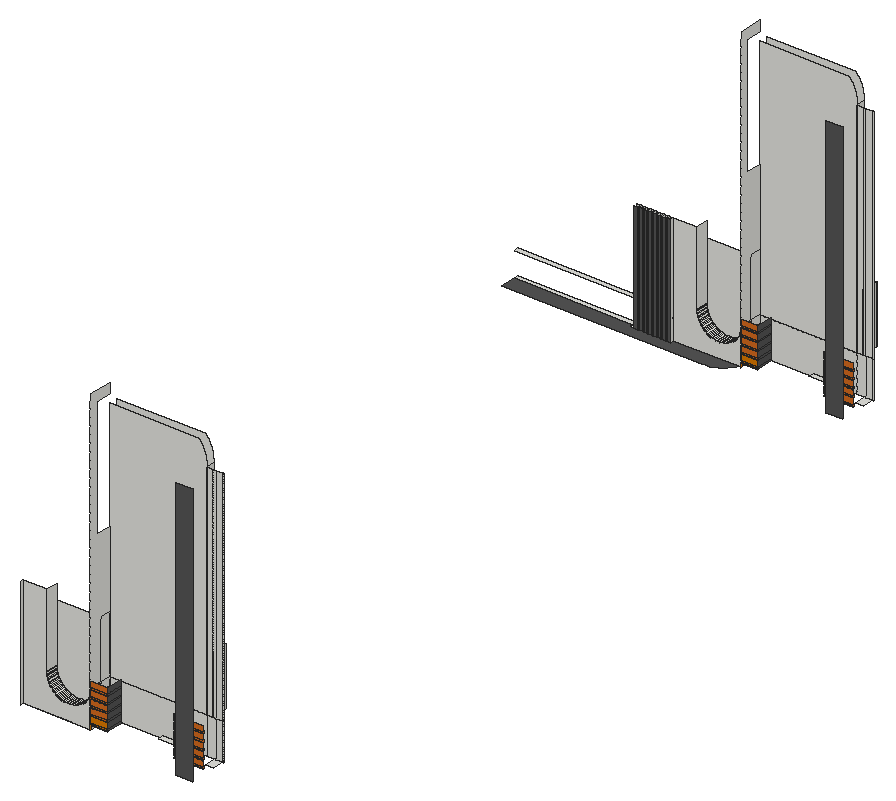
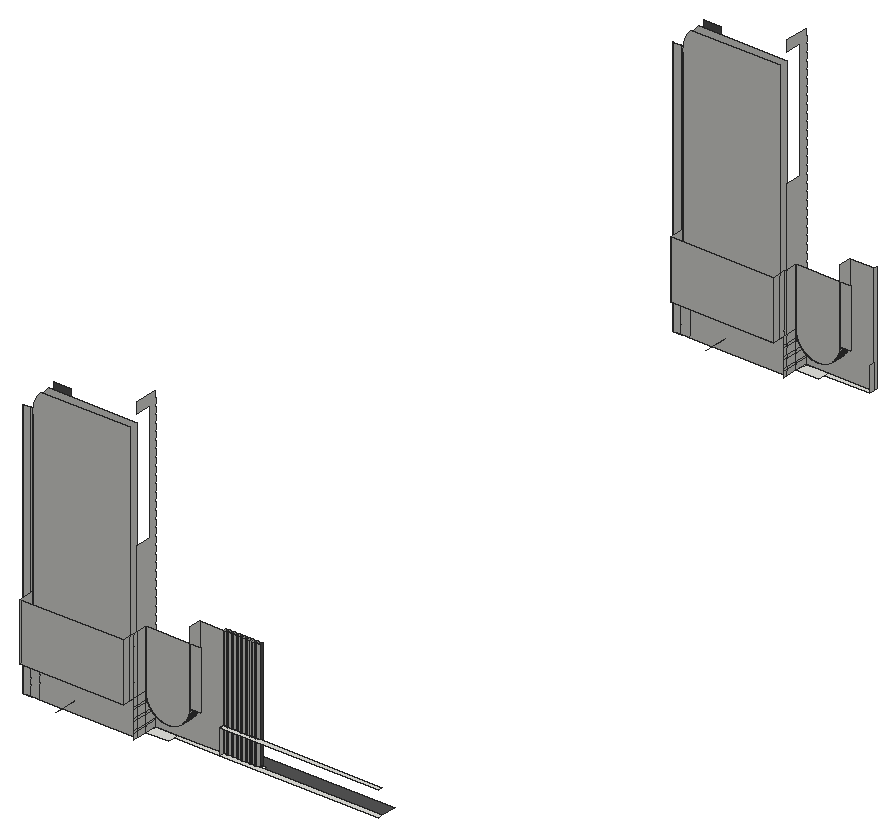
# SketchUp Ruby script. Lengths in inches.
U = 1.inch
M = Sketchup.active_model
def pt(a) = Geom::Point3d.new(a.map { |v| v * U })
def face(e, loops, mat)
  f = e.add_face(loops[0].map { |a| pt(a) })
  loops[1..].each { |l| e.add_face(l.map { |a| pt(a) }).erase! }
  f.material = f.back_material = mat if mat
  f
end
# faces: each face lists its corners as indices into pts; further lists are holes
def faces(e, pts, list, mat = nil) = list.each { |f| face(e, (f[0].is_a?(Array) ? f : [f]).map { |l| l.map { |i| pts[i] } }, mat) }
# xy, xz, yz: faces in a plane at the given z, y or x. An outline is a flat list of corners, or four numbers for a rectangle; further outlines are holes
def ring(l) = l.size == 4 ? [[l[0], l[1]], [l[2], l[1]], [l[2], l[3]], [l[0], l[3]]] : l.each_slice(2).to_a
def flat(e, list, mat, &to3) = list.each { |f| face(e, (f[0].is_a?(Array) ? f : [f]).map { |l| ring(l).map { |u, v| to3.(u, v) } }, mat) }
def xy(e, z, list, mat = nil) = flat(e, list, mat) { |x, y| [x, y, z] }
def xz(e, y, list, mat = nil) = flat(e, list, mat) { |x, z| [x, y, z] }
def yz(e, x, list, mat = nil) = flat(e, list, mat) { |y, z| [x, y, z] }
def lines(e, pts, list) = list.each { |a, b| e.add_line(pt(pts[a]), pt(pts[b])) }
# prism: a flat outline (further loops are holes) pulled along v
def prism(e, loops, v, mat = nil)
  f = face(e, loops, mat); d = Geom::Vector3d.new(v.map { |x| x * U })
  f.pushpull(f.normal.samedirection?(d) ? d.length : -d.length)
end
def box(e, o, s, mat = nil) = prism(e, [[o, [o[0] + s[0], o[1], o[2]], [o[0] + s[0], o[1] + s[1], o[2]], [o[0], o[1] + s[1], o[2]]]], [0, 0, s[2]], mat)
def at(x, y, z, deg = 0) = Geom::Transformation.translation(pt([x, y, z])) * Geom::Transformation.rotation(ORIGIN, Z_AXIS, deg.degrees)
def axes(o, x, y, z) = Geom::Transformation.new([*x, 0, *y, 0, *z, 0, *pt(o).to_a, 1])
def part(name) = M.definitions.add(name)
# library, detail: a bought-in or finely detailed component or shape, given as its bounding box
def library(name, o, s) = part(name).tap { |d| box(d.entities, o, s) }
def detail(e, o, s) = box(e.add_group.entities, o, s)
def put(e, d, t, mat = nil) = e.add_instance(d, t).tap { |i| i.material = mat if mat }
def group(e, t, mat = nil) = e.add_group.tap { |g| g.transformation = t; g.material = mat if mat }.entities
root = M.entities
M.materials.add("[0039_DarkOrange]").color = [219, 120, 0]
M.materials.add("[0041_Chocolate]").color = [210, 105, 30]
M.materials.add("[Color M06]").color = [84, 84, 84]
xy(root,141.26,[[2137,281.47,2177.59,285.84],[2177.59,281.47,2195.57,281.47,2196.33,283,2197.37,286.06,2198,289.23,2198.21,292.45,2177.59,292.45],[2195.57,281.47,2196.33,283,2197.37,286.06,2198,289.23,2198.21,292.45,2198.21,281.47],[2292.85,292.45,2299.64,302.46],[2026.42,972.36,2169.44,976.74],
  [2169.44,972.36,2210.03,976.74],[2210.03,972.36,2228.01,972.36,2228.77,973.89,2229.81,976.95,2230.4375,980.12,2230.65,983.34,2210.03,983.34],[2228.01,972.36,2228.77,973.89,2229.81,976.95,2230.4375,980.12,2230.65,983.34,2230.65,972.36],[2325.29,983.34,2332.08,993.35]])
xy(root,141.26,[[2026.42,958.64,2205.95,958.64,2209.17,958.86,2212.34,959.49,2215.4,960.52,2218.3,961.95,2220.98,963.75,2223.41,965.88,2225.54,968.31,2227.34,970.99,2228.01,972.36,2169.44,972.36,2169.44,969.24,2166.32,969.24,2166.32,972.36,2165.07,972.36,2165.07,969.24,2161.94,969.24,2161.94,972.36,2160.88,972.36,2160.88,969.24,2157.75,969.24,2157.75,972.36,2156.69,972.36,2156.69,969.24,2153.57,969.24,2153.57,972.36,2152.5,972.36,2152.5,969.24,2149.38,969.24,2149.38,972.36,2148.32,972.36,2148.32,969.24,2145.19,969.24,2145.19,972.36,2144.07,972.36,2144.07,969.24,2140.94,969.24,2140.94,972.36,2139.82,972.36,2139.82,969.24,2136.69,969.24,2136.69,972.36,2135.57,972.36,2135.57,969.24,2132.44,969.24,2132.44,972.36,2026.42,972.36]],"[Color M06]")
xy(root,145.27,[[2247.98,295.65,2273.17,300.34],[2280.42,986.55,2305.61,991.24]])
xy(root,145.27,[[2198.21,280.47,2213.6,281.47],[2230.65,971.36,2246.03,972.36]],"[0039_DarkOrange]")
xy(root,145.27,[[2273.17,280.47,2299.64,281.47],[2305.61,971.36,2332.08,972.36]],"[0041_Chocolate]")
xy(root,147.375,[[2198.21,280.47,2213.6,281.47],[2230.65,971.36,2246.03,972.36]],"[0039_DarkOrange]")
xy(root,147.375,[[2273.17,280.47,2299.64,281.47],[2305.61,971.36,2332.08,972.36]],"[0041_Chocolate]")
xy(root,152.33,[[2198.21,280.47,2213.6,281.47],[2230.65,971.36,2246.03,972.36]],"[0039_DarkOrange]")
xy(root,152.33,[[2273.17,280.47,2299.64,281.47],[2305.61,971.36,2332.08,972.36]],"[0041_Chocolate]")
xy(root,154.4375,[[2198.21,280.47,2213.6,281.47],[2273.17,280.47,2299.64,281.47],[2230.65,971.36,2246.03,972.36],[2305.61,971.36,2332.08,972.36]],"[0041_Chocolate]")
xy(root,159.39,[[2198.21,280.47,2213.6,281.47],[2273.17,280.47,2299.64,281.47],[2230.65,971.36,2246.03,972.36],[2305.61,971.36,2332.08,972.36]],"[0041_Chocolate]")
xy(root,161.5,[[2198.21,280.47,2213.6,281.47],[2273.17,280.47,2299.64,281.47],[2230.65,971.36,2246.03,972.36],[2305.61,971.36,2332.08,972.36]],"[0041_Chocolate]")
xy(root,163.7,[[2026.42,972.36,2169.44,976.74]])
xy(root,166.45,[[2198.21,280.47,2213.6,281.47],[2273.17,280.47,2299.64,281.47],[2230.65,971.36,2246.03,972.36],[2305.61,971.36,2332.08,972.36]],"[0041_Chocolate]")
xy(root,168.5625,[[2198.21,280.47,2213.6,281.47],[2273.17,280.47,2299.64,281.47],[2230.65,971.36,2246.03,972.36],[2305.61,971.36,2332.08,972.36]],"[0041_Chocolate]")
xy(root,173.52,[[2198.21,280.47,2213.6,281.47],[2273.17,280.47,2299.64,281.47],[2230.65,971.36,2246.03,972.36],[2305.61,971.36,2332.08,972.36]],"[0041_Chocolate]")
xy(root,174.51,[[2198.21,302.46,2285.18,310.27],[2285.18,302.46,2285.18,310.27,2198.21,310.27,2198.21,317.3125,2291.02,317.3125,2291.02,302.46],[2230.65,993.35,2317.62,1001.16],[2317.62,993.35,2317.62,1001.16,2230.65,1001.16,2230.65,1008.21,2323.46,1008.21,2323.46,993.35]])
xy(root,175.625,[[2198.21,280.47,2213.6,281.47],[2273.17,280.47,2299.64,281.47],[2230.65,971.36,2246.03,972.36],[2305.61,971.36,2332.08,972.36]],"[0041_Chocolate]")
xz(root,267.75,[[2285.18,141.3,2300.52,376.875]],"[Color M06]")
xz(root,280.47,[[2198.21,147.375,2213.6,152.33]],"[0039_DarkOrange]")
xz(root,280.47,[[2273.17,147.375,2299.64,152.33],[2198.21,154.4375,2213.6,159.39],[2273.17,154.4375,2299.64,159.39],[2198.21,161.5,2213.6,166.45],[2273.17,161.5,2299.64,166.45],
  [2198.21,168.5625,2213.6,173.52],[2273.17,168.5625,2299.64,173.52],[2198.21,175.625,2213.6,180.58],[2273.17,175.625,2299.64,180.58]],"[0041_Chocolate]")
xz(root,281.47,[[2137,141.26,2198.21,141.26,2198.21,174.51,2198.18,173.46,2198.1,172.42,2197.96,171.38,2197.77,170.36,2197.53,169.34,2197.23,168.33,2196.88,167.35,2196.48,166.38,2196.03,165.4375,2195.53,164.52,2194.99,163.625,2194.39,162.76,2193.76,161.93,2193.08,161.14,2192.36,160.38,2191.6,159.66,2190.8,158.98,2189.97,158.34,2189.11,157.75,2188.22,157.2,2187.3,156.7,2186.36,156.25,2185.39,155.85,2184.4,155.5,2183.4,155.21,2182.38,154.96,2181.35,154.77,2180.32,154.64,2179.27,154.55,2178.23,154.53,2177.18,154.55,2176.14,154.64,2175.1,154.77,2174.07,154.96,2173.05,155.21,2172.05,155.5,2171.07,155.85,2170.1,156.25,2169.15,156.7,2168.23,157.2,2167.34,157.75,2166.48,158.34,2165.65,158.98,2164.85,159.66,2164.1,160.38,2163.375,161.14,2162.7,161.93,2162.06,162.76,2161.47,163.625,2160.92,164.52,2160.42,165.4375,2159.97,166.38,2159.57,167.35,2159.22,168.33,2158.92,169.34,2158.68,170.36,2158.49,171.38,2158.35,172.42,2158.27,173.46,2158.24,174.51,2158.24,240.16,2137,240.16]])
xz(root,281.47,[[2198.21,145.27,2213.6,147.375]],"[0039_DarkOrange]")
xz(root,281.47,[[2273.17,145.27,2299.64,147.375],[2198.21,152.33,2213.6,154.4375],[2273.17,152.33,2299.64,154.4375],[2198.21,159.39,2213.6,161.5],[2273.17,159.39,2299.64,161.5],
  [2198.21,166.45,2213.6,168.5625],[2273.17,166.45,2299.64,168.5625],[2198.21,173.52,2213.6,175.625],[2273.17,173.52,2299.64,175.625]],"[0041_Chocolate]")
xz(root,292.45,[[2178.23,154.53,2179.27,154.55,2180.32,154.64,2181.35,154.77,2182.38,154.96,2183.4,155.21,2184.4,155.5,2185.39,155.85,2186.36,156.25,2187.3,156.7,2188.22,157.2,2189.11,157.75,2189.97,158.34,2190.8,158.98,2191.6,159.66,2192.36,160.38,2193.08,161.14,2193.76,161.93,2194.39,162.76,2194.99,163.625,2195.53,164.52,2196.03,165.4375,2196.48,166.38,2196.88,167.35,2197.23,168.33,2197.53,169.34,2197.77,170.36,2197.96,171.38,2198.1,172.42,2198.18,173.46,2198.21,174.51,2198.21,226.8,2158.24,226.8,2158.24,174.51,2158.27,173.46,2158.35,172.42,2158.49,171.38,2158.68,170.36,2158.92,169.34,2159.22,168.33,2159.57,167.35,2159.97,166.38,2160.42,165.4375,2160.92,164.52,2161.47,163.625,2162.06,162.76,2162.7,161.93,2163.375,161.14,2164.1,160.38,2164.85,159.66,2165.65,158.98,2166.48,158.34,2167.34,157.75,2168.23,157.2,2169.15,156.7,2170.1,156.25,2171.07,155.85,2172.05,155.5,2173.05,155.21,2174.07,154.96,2175.1,154.77,2176.14,154.64,2177.18,154.55],[2148.59,174.51,2158.24,226.8]])
xz(root,302.46,[[2198.21,141.26,2285.18,174.51],[2285.18,141.26,2293.73,174.51],[2293.73,141.26,2299.64,174.51],[2299.64,141.26,2300.52,174.51],[2198.21,174.51,2285.18,174.51,2285.18,376.875,2285.17,377.55,2285.14,378.22,2285.1,378.9,2285.04,379.57,2284.96,380.24,2284.86,380.9,2284.75,381.57,2284.62,382.23,2284.47,382.89,2284.3,383.54,2284.28,383.64,2284.12,384.19,2283.92,384.84,2283.7,385.47,2283.6,385.76,2283.47,386.11,2283.22,386.73,2282.95,387.35,2282.67,387.96,2282.37,388.57,2282.06,389.17,2281.73,389.76,2281.38,390.33,2281.02,390.9,2280.65,391.47,2280.26,392.02,2279.86,392.56,2279.4375,393.09,2279.4,393.14,2279.01,393.6,2278.5625,394.11,2278.1,394.61,2277.63,395.09,2277.46,395.26,2198.21,395.26],
  [2285.18,174.51,2291.02,374.14],[2291.02,174.51,2293.73,374.14],[2293.73,174.51,2299.64,374.14],[2299.64,174.51,2300.52,374.14]])
xz(root,310.27,[[2198.21,174.51,2198.21,395.26,2277.46,395.26,2277.63,395.09,2278.1,394.61,2278.5625,394.11,2279.01,393.6,2279.4,393.14,2279.4375,393.09,2279.86,392.56,2280.26,392.02,2280.65,391.47,2281.02,390.9,2281.38,390.33,2281.73,389.76,2282.06,389.17,2282.37,388.57,2282.67,387.96,2282.95,387.35,2283.22,386.73,2283.47,386.11,2283.6,385.76,2283.7,385.47,2283.92,384.84,2284.12,384.19,2284.28,383.64,2284.3,383.54,2284.47,382.89,2284.62,382.23,2284.75,381.57,2284.86,380.9,2284.96,380.24,2285.04,379.57,2285.1,378.9,2285.14,378.22,2285.17,377.55,2285.18,376.875,2285.18,174.51]])
xz(root,317.3125,[[2198.21,174.51,2291.02,226.8]])
xz(root,958.64,[[2317.62,141.3,2332.96,376.875]],"[Color M06]")
xz(root,969.24,[[2136.69,141.26,2139.82,240.16],[2140.94,141.26,2144.07,240.16],[2145.19,141.26,2148.32,240.16],[2149.38,141.26,2152.5,240.16],[2153.57,141.26,2156.69,240.16],
  [2157.75,141.26,2160.88,240.16],[2161.94,141.26,2165.07,240.16],[2166.32,141.26,2169.44,240.16]],"[Color M06]")
xz(root,971.36,[[2230.65,147.375,2246.03,152.33]],"[0039_DarkOrange]")
xz(root,971.36,[[2305.61,147.375,2332.08,152.33],[2230.65,154.4375,2246.03,159.39],[2305.61,154.4375,2332.08,159.39],[2230.65,161.5,2246.03,166.45],[2305.61,161.5,2332.08,166.45],
  [2230.65,168.5625,2246.03,173.52],[2305.61,168.5625,2332.08,173.52],[2230.65,175.625,2246.03,180.58],[2305.61,175.625,2332.08,180.58]],"[0041_Chocolate]")
xz(root,972.36,[[2136.69,141.26,2139.82,163.7],[2139.82,141.26,2140.94,163.7],[2140.94,141.26,2144.07,163.7],[2144.07,141.26,2145.19,163.7],[2145.19,141.26,2148.32,163.7],
  [2148.32,141.26,2149.38,163.7],[2149.38,141.26,2152.5,163.7],[2152.5,141.26,2153.57,163.7],[2153.57,141.26,2156.69,163.7],[2156.69,141.26,2157.75,163.7],
  [2157.75,141.26,2160.88,163.7],[2160.88,141.26,2161.94,163.7],[2161.94,141.26,2165.07,163.7],[2165.07,141.26,2166.32,163.7],[2166.32,141.26,2169.44,163.7],
  [2169.44,141.26,2230.65,141.26,2230.65,174.51,2230.62,173.46,2230.54,172.42,2230.4,171.38,2230.21,170.36,2229.97,169.34,2229.67,168.33,2229.32,167.35,2228.92,166.38,2228.47,165.4375,2227.97,164.52,2227.42,163.625,2226.83,162.76,2226.19,161.93,2225.52,161.14,2224.8,160.38,2224.04,159.66,2223.24,158.98,2222.41,158.34,2221.55,157.75,2220.66,157.2,2219.74,156.7,2218.79,156.25,2217.83,155.85,2216.84,155.5,2215.84,155.21,2214.82,154.96,2213.79,154.77,2212.75,154.64,2211.71,154.55,2210.66,154.53,2209.62,154.55,2208.58,154.64,2207.54,154.77,2206.51,154.96,2205.49,155.21,2204.49,155.5,2203.5,155.85,2202.54,156.25,2201.59,156.7,2200.67,157.2,2199.78,157.75,2198.92,158.34,2198.09,158.98,2197.29,159.66,2196.53,160.38,2195.8125,161.14,2195.13,161.93,2194.5,162.76,2193.9,163.625,2193.36,164.52,2192.86,165.4375,2192.41,166.38,2192.01,167.35,2191.66,168.33,2191.36,169.34,2191.12,170.36,2190.93,171.38,2190.79,172.42,2190.71,173.46,2190.68,174.51,2190.68,240.16,2169.44,240.16],[2136.69,163.7,2139.82,240.16],[2140.94,163.7,2144.07,240.16],[2145.19,163.7,2148.32,240.16],[2149.38,163.7,2152.5,240.16],
  [2153.57,163.7,2156.69,240.16],[2157.75,163.7,2160.88,240.16],[2161.94,163.7,2165.07,240.16],[2166.32,163.7,2169.44,240.16]])
xz(root,972.36,[[2230.65,145.27,2246.03,147.375]],"[0039_DarkOrange]")
xz(root,972.36,[[2305.61,145.27,2332.08,147.375],[2230.65,152.33,2246.03,154.4375],[2305.61,152.33,2332.08,154.4375],[2230.65,159.39,2246.03,161.5],[2305.61,159.39,2332.08,161.5],
  [2230.65,166.45,2246.03,168.5625],[2305.61,166.45,2332.08,168.5625],[2230.65,173.52,2246.03,175.625],[2305.61,173.52,2332.08,175.625]],"[0041_Chocolate]")
xz(root,983.34,[[2210.66,154.53,2211.71,154.55,2212.75,154.64,2213.79,154.77,2214.82,154.96,2215.84,155.21,2216.84,155.5,2217.83,155.85,2218.79,156.25,2219.74,156.7,2220.66,157.2,2221.55,157.75,2222.41,158.34,2223.24,158.98,2224.04,159.66,2224.8,160.38,2225.52,161.14,2226.19,161.93,2226.83,162.76,2227.42,163.625,2227.97,164.52,2228.47,165.4375,2228.92,166.38,2229.32,167.35,2229.67,168.33,2229.97,169.34,2230.21,170.36,2230.4,171.38,2230.54,172.42,2230.62,173.46,2230.65,174.51,2230.65,226.8,2190.68,226.8,2190.68,174.51,2190.71,173.46,2190.79,172.42,2190.93,171.38,2191.12,170.36,2191.36,169.34,2191.66,168.33,2192.01,167.35,2192.41,166.38,2192.86,165.4375,2193.36,164.52,2193.9,163.625,2194.5,162.76,2195.13,161.93,2195.8125,161.14,2196.53,160.38,2197.29,159.66,2198.09,158.98,2198.92,158.34,2199.78,157.75,2200.67,157.2,2201.59,156.7,2202.54,156.25,2203.5,155.85,2204.49,155.5,2205.49,155.21,2206.51,154.96,2207.54,154.77,2208.58,154.64,2209.62,154.55],[2181.03,174.51,2190.68,226.8]])
xz(root,993.35,[[2230.65,141.26,2317.62,174.51],[2317.62,141.26,2326.17,174.51],[2326.17,141.26,2332.08,174.51],[2332.08,141.26,2332.96,174.51],[2230.65,174.51,2317.62,174.51,2317.62,376.875,2317.61,377.55,2317.58,378.22,2317.54,378.9,2317.48,379.57,2317.4,380.24,2317.3,380.9,2317.19,381.57,2317.05,382.23,2316.9,382.89,2316.74,383.54,2316.71,383.64,2316.56,384.19,2316.36,384.84,2316.14,385.47,2316.03,385.76,2315.91,386.11,2315.66,386.73,2315.39,387.35,2315.11,387.96,2314.81,388.57,2314.49,389.17,2314.17,389.76,2313.82,390.33,2313.46,390.9,2313.09,391.47,2312.7,392.02,2312.29,392.56,2311.875,393.09,2311.84,393.14,2311.44,393.6,2311,394.11,2310.54,394.61,2310.07,395.09,2309.9,395.26,2230.65,395.26],
  [2317.62,174.51,2323.46,374.14],[2323.46,174.51,2326.17,374.14],[2326.17,174.51,2332.08,374.14],[2332.08,174.51,2332.96,374.14]])
xz(root,1001.16,[[2230.65,174.51,2230.65,395.26,2309.9,395.26,2310.07,395.09,2310.54,394.61,2311,394.11,2311.44,393.6,2311.84,393.14,2311.875,393.09,2312.29,392.56,2312.7,392.02,2313.09,391.47,2313.46,390.9,2313.82,390.33,2314.17,389.76,2314.49,389.17,2314.81,388.57,2315.11,387.96,2315.39,387.35,2315.66,386.73,2315.91,386.11,2316.03,385.76,2316.14,385.47,2316.36,384.84,2316.56,384.19,2316.71,383.64,2316.74,383.54,2316.9,382.89,2317.05,382.23,2317.19,381.57,2317.3,380.9,2317.4,380.24,2317.48,379.57,2317.54,378.9,2317.58,378.22,2317.61,377.55,2317.62,376.875,2317.62,174.51]])
xz(root,1008.21,[[2230.65,174.51,2323.46,226.8]])
yz(root,2137,[[278.34,141.26,281.47,240.16],[281.47,141.26,285.84,163.7]])
yz(root,2139.82,[[969.24,141.26,972.36,240.16]])
yz(root,2140.94,[[969.24,141.26,972.36,240.16]])
yz(root,2144.07,[[969.24,141.26,972.36,240.16]])
yz(root,2145.19,[[969.24,141.26,972.36,240.16]])
yz(root,2148.32,[[969.24,141.26,972.36,240.16]])
yz(root,2149.38,[[969.24,141.26,972.36,240.16]])
yz(root,2152.5,[[969.24,141.26,972.36,240.16]])
yz(root,2153.57,[[969.24,141.26,972.36,240.16]])
yz(root,2156.69,[[969.24,141.26,972.36,240.16]])
yz(root,2157.75,[[969.24,141.26,972.36,240.16]])
yz(root,2158.24,[[281.47,174.51,292.45,240.16]])
yz(root,2160.88,[[969.24,141.26,972.36,240.16]])
yz(root,2161.94,[[969.24,141.26,972.36,240.16]])
yz(root,2165.07,[[969.24,141.26,972.36,240.16]])
yz(root,2166.32,[[969.24,141.26,972.36,240.16]])
yz(root,2169.44,[[969.24,141.26,972.36,240.16],[972.36,141.26,976.74,163.7]])
yz(root,2190.68,[[972.36,174.51,983.34,240.16]])
yz(root,2198.21,[[281.47,141.26,292.45,146.14],[292.45,141.26,302.46,146.14],[302.46,141.26,305.58,146.14],[281.47,146.14,292.45,148.26],[292.45,146.14,302.46,148.26],
  [302.46,146.14,305.58,148.26],[281.47,148.26,292.45,155.64],[292.45,148.26,302.46,155.64],[302.46,148.26,305.58,155.64],[281.47,155.64,292.45,157.76],
  [292.45,155.64,302.46,157.76],[302.46,155.64,305.58,157.76],[281.47,157.76,292.45,165.14],[292.45,157.76,302.46,165.14],[302.46,157.76,305.58,165.14],
  [281.47,165.14,292.45,167.26],[292.45,165.14,302.46,167.26],[302.46,165.14,305.58,167.26],[281.47,167.26,292.45,174.51],[292.45,167.26,302.46,174.51],
  [302.46,167.26,305.58,174.51],[281.47,174.51,281.47,175.625,280.47,175.625,280.47,180.58,281.47,180.58,281.47,182.6875,280.47,182.6875,280.47,187.64,281.47,187.64,281.47,189.75,280.47,189.75,280.47,194.7,281.47,194.7,281.47,196.8125,280.47,196.8125,280.47,201.77,281.47,201.77,281.47,203.875,280.47,203.875,280.47,208.83,281.47,208.83,281.47,210.9375,280.47,210.9375,280.47,215.89,281.47,215.89,281.47,218,280.47,218,280.47,222.95,281.47,222.95,281.47,225.0625,280.47,225.0625,280.47,230.02,281.47,230.02,281.47,232.125,280.47,232.125,280.47,237.08,281.47,237.08,281.47,239.1875,280.47,239.1875,280.47,244.14,281.47,244.14,281.47,246.25,280.47,246.25,280.47,251.2,281.47,251.2,281.47,253.3125,280.47,253.3125,280.47,258.27,281.47,258.27,281.47,260.375,280.47,260.375,280.47,265.33,281.47,265.33,281.47,267.4375,280.47,267.4375,280.47,272.39,281.47,272.39,281.47,274.5,280.47,274.5,280.47,279.45,281.47,279.45,281.47,281.5625,280.47,281.5625,280.47,286.52,281.47,286.52,281.47,288.625,280.47,288.625,280.47,293.58,281.47,293.58,281.47,295.6875,280.47,295.6875,280.47,300.64,281.47,300.64,281.47,302.75,280.47,302.75,280.47,307.7,281.47,307.7,281.47,309.8125,280.47,309.8125,280.47,314.77,281.47,314.77,281.47,316.875,280.47,316.875,280.47,321.83,281.47,321.83,281.47,323.9375,280.47,323.9375,280.47,328.89,281.47,328.89,281.47,331,280.47,331,280.47,335.95,281.47,335.95,281.47,338.0625,280.47,338.0625,280.47,343.02,281.47,343.02,281.47,345.125,280.47,345.125,280.47,350.08,281.47,350.08,281.47,352.1875,280.47,352.1875,280.47,357.14,281.47,357.14,281.47,359.25,280.47,359.25,280.47,364.2,281.47,364.2,281.47,366.3125,280.47,366.3125,280.47,371.27,281.47,371.27,281.47,373.1875,280.47,373.1875,280.47,378.14,281.47,378.14,281.47,380.0625,280.47,380.0625,280.47,385.02,281.47,385.02,281.47,386.9375,280.47,386.9375,280.47,391.89,281.47,391.89,281.47,393.8125,280.47,393.8125,280.47,398.77,281.47,398.77,281.47,400.6875,280.47,400.6875,280.47,405.64,281.47,405.64,281.47,411.82,302.46,411.82,302.46,402.64,287.95,402.64,287.95,295.72,302.0625,295.72,302.0625,226.8,292.45,226.8,292.45,174.51],[292.45,174.51,302.46,226.8],[302.46,174.51,305.58,226.8],[305.58,174.51,310.27,226.8],
  [310.27,174.51,317.3125,226.8]])
yz(root,2198.21,[[280.47,141.26,281.47,145.27],[280.47,147.375,281.47,148.26],[280.47,148.26,281.47,152.33]],"[0039_DarkOrange]")
yz(root,2198.21,[[280.47,154.4375,281.47,155.64],[280.47,155.64,281.47,157.76],[280.47,157.76,281.47,159.39],[280.47,161.5,281.47,165.14],[280.47,165.14,281.47,166.45],
  [280.47,168.5625,281.47,173.52]],"[0041_Chocolate]")
yz(root,2213.6,[[281.47,145.27,295.65,147.375],[280.47,147.375,295.65,152.33],[281.47,152.33,295.65,154.4375],[280.47,154.4375,295.65,159.39],[281.47,159.39,295.65,161.5],
  [280.47,161.5,295.65,166.45],[281.47,166.45,295.65,168.5625],[280.47,168.5625,295.65,173.52],[281.47,173.52,295.65,175.625],[280.47,175.625,295.65,180.58]],"[Color M06]")
yz(root,2230.65,[[972.36,141.26,983.34,146.14],[983.34,141.26,993.35,146.14],[993.35,141.26,996.48,146.14],[972.36,146.14,983.34,148.26],[983.34,146.14,993.35,148.26],
  [993.35,146.14,996.48,148.26],[972.36,148.26,983.34,155.64],[983.34,148.26,993.35,155.64],[993.35,148.26,996.48,155.64],[972.36,155.64,983.34,157.76],
  [983.34,155.64,993.35,157.76],[993.35,155.64,996.48,157.76],[972.36,157.76,983.34,165.14],[983.34,157.76,993.35,165.14],[993.35,157.76,996.48,165.14],
  [972.36,165.14,983.34,167.26],[983.34,165.14,993.35,167.26],[993.35,165.14,996.48,167.26],[972.36,167.26,983.34,174.51],[983.34,167.26,993.35,174.51],
  [993.35,167.26,996.48,174.51],[972.36,174.51,972.36,175.625,971.36,175.625,971.36,180.58,972.36,180.58,972.36,182.6875,971.36,182.6875,971.36,187.64,972.36,187.64,972.36,189.75,971.36,189.75,971.36,194.7,972.36,194.7,972.36,196.8125,971.36,196.8125,971.36,201.77,972.36,201.77,972.36,203.875,971.36,203.875,971.36,208.83,972.36,208.83,972.36,210.9375,971.36,210.9375,971.36,215.89,972.36,215.89,972.36,218,971.36,218,971.36,222.95,972.36,222.95,972.36,225.0625,971.36,225.0625,971.36,230.02,972.36,230.02,972.36,232.125,971.36,232.125,971.36,237.08,972.36,237.08,972.36,239.1875,971.36,239.1875,971.36,244.14,972.36,244.14,972.36,246.25,971.36,246.25,971.36,251.2,972.36,251.2,972.36,253.3125,971.36,253.3125,971.36,258.27,972.36,258.27,972.36,260.375,971.36,260.375,971.36,265.33,972.36,265.33,972.36,267.4375,971.36,267.4375,971.36,272.39,972.36,272.39,972.36,274.5,971.36,274.5,971.36,279.45,972.36,279.45,972.36,281.5625,971.36,281.5625,971.36,286.52,972.36,286.52,972.36,288.625,971.36,288.625,971.36,293.58,972.36,293.58,972.36,295.6875,971.36,295.6875,971.36,300.64,972.36,300.64,972.36,302.75,971.36,302.75,971.36,307.7,972.36,307.7,972.36,309.8125,971.36,309.8125,971.36,314.77,972.36,314.77,972.36,316.875,971.36,316.875,971.36,321.83,972.36,321.83,972.36,323.9375,971.36,323.9375,971.36,328.89,972.36,328.89,972.36,331,971.36,331,971.36,335.95,972.36,335.95,972.36,338.0625,971.36,338.0625,971.36,343.02,972.36,343.02,972.36,345.125,971.36,345.125,971.36,350.08,972.36,350.08,972.36,352.1875,971.36,352.1875,971.36,357.14,972.36,357.14,972.36,359.25,971.36,359.25,971.36,364.2,972.36,364.2,972.36,366.3125,971.36,366.3125,971.36,371.27,972.36,371.27,972.36,373.1875,971.36,373.1875,971.36,378.14,972.36,378.14,972.36,380.0625,971.36,380.0625,971.36,385.02,972.36,385.02,972.36,386.9375,971.36,386.9375,971.36,391.89,972.36,391.89,972.36,393.8125,971.36,393.8125,971.36,398.77,972.36,398.77,972.36,400.6875,971.36,400.6875,971.36,405.64,972.36,405.64,972.36,411.82,993.35,411.82,993.35,402.64,978.84,402.64,978.84,295.72,992.96,295.72,992.96,226.8,983.34,226.8,983.34,174.51],[983.34,174.51,993.35,226.8],[993.35,174.51,996.48,226.8],[996.48,174.51,1001.16,226.8],
  [1001.16,174.51,1008.21,226.8]])
yz(root,2230.65,[[971.36,141.26,972.36,145.27],[971.36,147.375,972.36,148.26],[971.36,148.26,972.36,152.33]],"[0039_DarkOrange]")
yz(root,2230.65,[[971.36,154.4375,972.36,155.64],[971.36,155.64,972.36,157.76],[971.36,157.76,972.36,159.39],[971.36,161.5,972.36,165.14],[971.36,165.14,972.36,166.45],
  [971.36,168.5625,972.36,173.52]],"[0041_Chocolate]")
yz(root,2246.03,[[972.36,145.27,986.55,147.375],[971.36,147.375,986.55,152.33],[972.36,152.33,986.55,154.4375],[971.36,154.4375,986.55,159.39],[972.36,159.39,986.55,161.5],
  [971.36,161.5,986.55,166.45],[972.36,166.45,986.55,168.5625],[971.36,168.5625,986.55,173.52],[972.36,173.52,986.55,175.625],[971.36,175.625,986.55,180.58]],"[Color M06]")
yz(root,2273.17,[[281.47,145.27,295.65,147.375],[280.47,147.375,295.65,152.33],[281.47,152.33,295.65,154.4375],[280.47,154.4375,295.65,159.39],[281.47,159.39,295.65,161.5],
  [280.47,161.5,295.65,166.45],[281.47,166.45,295.65,168.5625],[280.47,168.5625,295.65,173.52],[281.47,173.52,295.65,175.625],[280.47,175.625,295.65,180.58]],"[Color M06]")
yz(root,2285.18,[[302.46,174.51,310.27,374.14]])
yz(root,2291.02,[[302.46,174.51,317.3125,226.8]])
yz(root,2305.61,[[972.36,145.27,986.55,147.375],[971.36,147.375,986.55,152.33],[972.36,152.33,986.55,154.4375],[971.36,154.4375,986.55,159.39],[972.36,159.39,986.55,161.5],
  [971.36,161.5,986.55,166.45],[972.36,166.45,986.55,168.5625],[971.36,168.5625,986.55,173.52],[972.36,173.52,986.55,175.625],[971.36,175.625,986.55,180.58]],"[Color M06]")
yz(root,2317.62,[[993.35,174.51,1001.16,374.14]])
yz(root,2323.46,[[993.35,174.51,1008.21,226.8]])
p = [[2178.23,292.45,154.53],[2177.18,292.45,154.55],[2177.18,281.47,154.55],[2178.23,281.47,154.53],[2179.27,292.45,154.55],[2179.27,281.47,154.55],
  [2210.66,983.34,154.53],[2209.62,983.34,154.55],[2209.62,972.36,154.55],[2210.66,972.36,154.53],[2211.71,983.34,154.55],[2211.71,972.36,154.55],
  [2176.14,292.45,154.64],[2175.1,292.45,154.77],[2175.1,281.47,154.77],[2176.14,281.47,154.64],[2180.32,292.45,154.64],[2180.32,281.47,154.64],
  [2181.35,292.45,154.77],[2181.35,281.47,154.77],[2208.58,983.34,154.64],[2207.54,983.34,154.77],[2207.54,972.36,154.77],[2208.58,972.36,154.64],
  [2212.75,983.34,154.64],[2212.75,972.36,154.64],[2213.79,983.34,154.77],[2213.79,972.36,154.77],[2174.07,292.45,154.96],[2174.07,281.47,154.96],
  [2182.38,292.45,154.96],[2182.38,281.47,154.96],[2206.51,983.34,154.96],[2206.51,972.36,154.96],[2214.82,983.34,154.96],[2214.82,972.36,154.96],
  [2173.05,292.45,155.21],[2173.05,281.47,155.21],[2183.4,292.45,155.21],[2183.4,281.47,155.21],[2205.49,983.34,155.21],[2205.49,972.36,155.21],
  [2215.84,983.34,155.21],[2215.84,972.36,155.21],[2172.05,292.45,155.5],[2172.05,281.47,155.5],[2184.4,292.45,155.5],[2184.4,281.47,155.5],
  [2204.49,983.34,155.5],[2204.49,972.36,155.5],[2216.84,983.34,155.5],[2216.84,972.36,155.5],[2171.07,292.45,155.85],[2171.07,281.47,155.85],
  [2185.39,292.45,155.85],[2185.39,281.47,155.85],[2203.5,983.34,155.85],[2203.5,972.36,155.85],[2217.83,983.34,155.85],[2217.83,972.36,155.85],
  [2170.1,292.45,156.25],[2170.1,281.47,156.25],[2186.36,292.45,156.25],[2186.36,281.47,156.25],[2202.54,983.34,156.25],[2202.54,972.36,156.25],
  [2218.79,983.34,156.25],[2218.79,972.36,156.25],[2169.15,292.45,156.7],[2169.15,281.47,156.7],[2187.3,292.45,156.7],[2187.3,281.47,156.7],
  [2201.59,983.34,156.7],[2201.59,972.36,156.7],[2219.74,983.34,156.7],[2219.74,972.36,156.7],[2168.23,292.45,157.2],[2168.23,281.47,157.2],
  [2188.22,292.45,157.2],[2188.22,281.47,157.2],[2200.67,983.34,157.2],[2200.67,972.36,157.2],[2220.66,983.34,157.2],[2220.66,972.36,157.2],
  [2167.34,292.45,157.75],[2167.34,281.47,157.75],[2189.11,292.45,157.75],[2189.11,281.47,157.75],[2199.78,983.34,157.75],[2199.78,972.36,157.75],
  [2221.55,983.34,157.75],[2221.55,972.36,157.75],[2166.48,292.45,158.34],[2166.48,281.47,158.34],[2189.97,292.45,158.34],[2189.97,281.47,158.34],
  [2198.92,983.34,158.34],[2198.92,972.36,158.34],[2222.41,983.34,158.34],[2222.41,972.36,158.34],[2165.65,292.45,158.98],[2165.65,281.47,158.98],
  [2190.8,292.45,158.98],[2190.8,281.47,158.98],[2198.09,983.34,158.98],[2198.09,972.36,158.98],[2223.24,983.34,158.98],[2223.24,972.36,158.98],
  [2164.85,292.45,159.66],[2164.85,281.47,159.66],[2191.6,292.45,159.66],[2191.6,281.47,159.66],[2197.29,983.34,159.66],[2197.29,972.36,159.66],
  [2224.04,983.34,159.66],[2224.04,972.36,159.66],[2164.1,292.45,160.38],[2164.1,281.47,160.38],[2192.36,292.45,160.38],[2192.36,281.47,160.38],
  [2196.53,983.34,160.38],[2196.53,972.36,160.38],[2224.8,983.34,160.38],[2224.8,972.36,160.38],[2163.375,292.45,161.14],[2163.375,281.47,161.14],
  [2193.08,292.45,161.14],[2193.08,281.47,161.14],[2195.8125,983.34,161.14],[2195.8125,972.36,161.14],[2225.52,983.34,161.14],[2225.52,972.36,161.14],
  [2162.7,292.45,161.93],[2162.7,281.47,161.93],[2193.76,292.45,161.93],[2193.76,281.47,161.93],[2195.13,983.34,161.93],[2195.13,972.36,161.93],
  [2226.19,983.34,161.93],[2226.19,972.36,161.93],[2162.06,292.45,162.76],[2162.06,281.47,162.76],[2194.39,292.45,162.76],[2194.39,281.47,162.76],
  [2194.5,983.34,162.76],[2194.5,972.36,162.76],[2226.83,983.34,162.76],[2226.83,972.36,162.76],[2161.47,292.45,163.625],[2161.47,281.47,163.625],
  [2194.99,292.45,163.625],[2194.99,281.47,163.625],[2193.9,983.34,163.625],[2193.9,972.36,163.625],[2227.42,983.34,163.625],[2227.42,972.36,163.625],
  [2160.92,292.45,164.52],[2160.92,281.47,164.52],[2195.53,292.45,164.52],[2195.53,281.47,164.52],[2193.36,983.34,164.52],[2193.36,972.36,164.52],
  [2227.97,983.34,164.52],[2227.97,972.36,164.52],[2160.42,292.45,165.4375],[2160.42,281.47,165.4375],[2196.03,292.45,165.4375],[2196.03,281.47,165.4375],
  [2192.86,983.34,165.4375],[2192.86,972.36,165.4375],[2228.47,983.34,165.4375],[2228.47,972.36,165.4375],[2159.97,292.45,166.38],[2159.97,281.47,166.38],
  [2196.48,292.45,166.38],[2196.48,281.47,166.38],[2192.41,983.34,166.38],[2192.41,972.36,166.38],[2228.92,983.34,166.38],[2228.92,972.36,166.38],
  [2159.57,292.45,167.35],[2159.57,281.47,167.35],[2196.88,292.45,167.35],[2196.88,281.47,167.35],[2192.01,983.34,167.35],[2192.01,972.36,167.35],
  [2229.32,983.34,167.35],[2229.32,972.36,167.35],[2159.22,292.45,168.33],[2159.22,281.47,168.33],[2197.23,292.45,168.33],[2197.23,281.47,168.33],
  [2191.66,983.34,168.33],[2191.66,972.36,168.33],[2229.67,983.34,168.33],[2229.67,972.36,168.33],[2158.92,292.45,169.34],[2158.92,281.47,169.34],
  [2197.53,292.45,169.34],[2197.53,281.47,169.34],[2191.36,983.34,169.34],[2191.36,972.36,169.34],[2229.97,983.34,169.34],[2229.97,972.36,169.34],
  [2158.68,292.45,170.36],[2158.68,281.47,170.36],[2197.77,292.45,170.36],[2197.77,281.47,170.36],[2191.12,983.34,170.36],[2191.12,972.36,170.36],
  [2230.21,983.34,170.36],[2230.21,972.36,170.36],[2158.49,292.45,171.38],[2158.49,281.47,171.38],[2197.96,292.45,171.38],[2197.96,281.47,171.38],
  [2190.93,983.34,171.38],[2190.93,972.36,171.38],[2230.4,983.34,171.38],[2230.4,972.36,171.38],[2158.35,292.45,172.42],[2158.35,281.47,172.42],
  [2198.1,292.45,172.42],[2198.1,281.47,172.42],[2190.79,983.34,172.42],[2190.79,972.36,172.42],[2230.54,983.34,172.42],[2230.54,972.36,172.42],
  [2158.27,292.45,173.46],[2158.27,281.47,173.46],[2198.18,292.45,173.46],[2198.18,281.47,173.46],[2190.71,983.34,173.46],[2190.71,972.36,173.46],
  [2230.62,983.34,173.46],[2230.62,972.36,173.46],[2158.24,292.45,174.51],[2158.24,281.47,174.51],[2198.21,292.45,174.51],[2198.21,281.47,174.51],
  [2190.68,983.34,174.51],[2190.68,972.36,174.51],[2230.65,983.34,174.51],[2230.65,972.36,174.51],[2238.76,321.34,165.14],[2238.76,343.15,165.14],
  [2271.2,1012.23,165.14],[2271.2,1034.04,165.14]]
faces(root,p,[[0,1,2,3],[4,0,3,5],[6,7,8,9],[10,6,9,11],[12,13,14,15],[1,12,15,2],[16,4,5,17],[18,16,17,19],
  [20,21,22,23],[7,20,23,8],[24,10,11,25],[26,24,25,27],[13,28,29,14],[30,18,19,31],[21,32,33,22],[34,26,27,35],
  [28,36,37,29],[38,30,31,39],[32,40,41,33],[42,34,35,43],[36,44,45,37],[46,38,39,47],[40,48,49,41],[50,42,43,51],
  [44,52,53,45],[54,46,47,55],[48,56,57,49],[58,50,51,59],[52,60,61,53],[62,54,55,63],[56,64,65,57],[66,58,59,67],
  [60,68,69,61],[70,62,63,71],[64,72,73,65],[74,66,67,75],[68,76,77,69],[78,70,71,79],[72,80,81,73],[82,74,75,83],
  [76,84,85,77],[86,78,79,87],[80,88,89,81],[90,82,83,91],[84,92,93,85],[94,86,87,95],[88,96,97,89],[98,90,91,99],
  [92,100,101,93],[102,94,95,103],[96,104,105,97],[106,98,99,107],[100,108,109,101],[110,102,103,111],[104,112,113,105],[114,106,107,115],
  [108,116,117,109],[118,110,111,119],[112,120,121,113],[122,114,115,123],[116,124,125,117],[126,118,119,127],[120,128,129,121],[130,122,123,131],
  [124,132,133,125],[134,126,127,135],[128,136,137,129],[138,130,131,139],[132,140,141,133],[142,134,135,143],[136,144,145,137],[146,138,139,147],
  [140,148,149,141],[150,142,143,151],[144,152,153,145],[154,146,147,155],[148,156,157,149],[158,150,151,159],[152,160,161,153],[162,154,155,163],
  [156,164,165,157],[166,158,159,167],[160,168,169,161],[170,162,163,171],[164,172,173,165],[174,166,167,175],[168,176,177,169],[178,170,171,179],
  [172,180,181,173],[182,174,175,183],[176,184,185,177],[186,178,179,187],[180,188,189,181],[190,182,183,191],[184,192,193,185],[194,186,187,195],
  [188,196,197,189],[198,190,191,199],[192,200,201,193],[202,194,195,203],[196,204,205,197],[206,198,199,207],[200,208,209,201],[210,202,203,211],
  [204,212,213,205],[214,206,207,215],[208,216,217,209],[218,210,211,219],[212,220,221,213],[222,214,215,223],[216,224,225,217],[226,218,219,227],
  [220,228,229,221],[230,222,223,231],[224,232,233,225],[234,226,227,235],[228,236,237,229],[238,230,231,239],[232,240,241,233],[242,234,235,243]])
lines(root,p,[[244,245],[246,247]])
